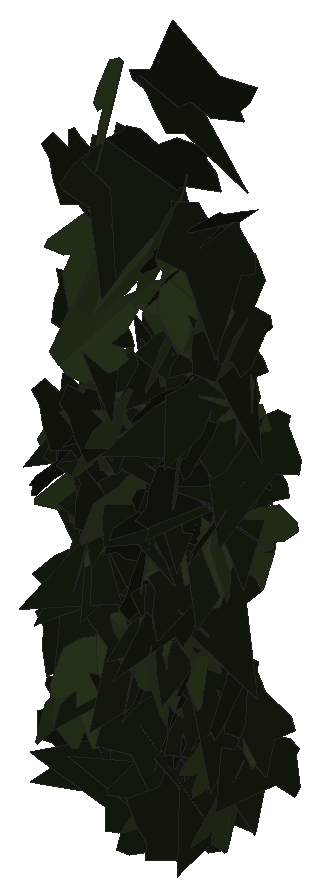
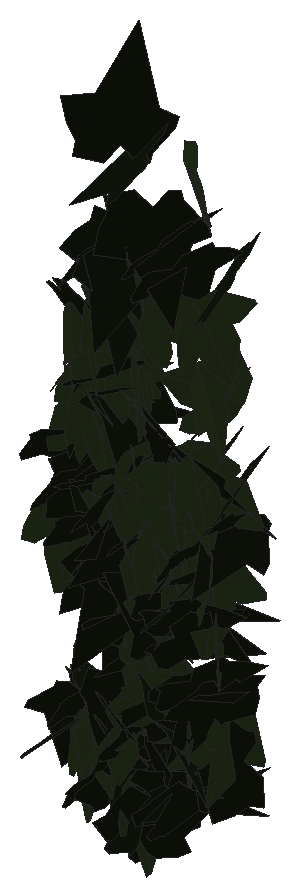
# SketchUp Ruby script. Lengths in inches.
U = 1.inch
M = Sketchup.active_model
def pt(a) = Geom::Point3d.new(a.map { |v| v * U })
def face(e, loops, mat)
  f = e.add_face(loops[0].map { |a| pt(a) })
  loops[1..].each { |l| e.add_face(l.map { |a| pt(a) }).erase! }
  f.material = f.back_material = mat if mat
  f
end
# faces: each face lists its corners as indices into pts; further lists are holes
def faces(e, pts, list, mat = nil) = list.each { |f| face(e, (f[0].is_a?(Array) ? f : [f]).map { |l| l.map { |i| pts[i] } }, mat) }
# xy, xz, yz: faces in a plane at the given z, y or x. An outline is a flat list of corners, or four numbers for a rectangle; further outlines are holes
def ring(l) = l.size == 4 ? [[l[0], l[1]], [l[2], l[1]], [l[2], l[3]], [l[0], l[3]]] : l.each_slice(2).to_a
def flat(e, list, mat, &to3) = list.each { |f| face(e, (f[0].is_a?(Array) ? f : [f]).map { |l| ring(l).map { |u, v| to3.(u, v) } }, mat) }
def xy(e, z, list, mat = nil) = flat(e, list, mat) { |x, y| [x, y, z] }
def xz(e, y, list, mat = nil) = flat(e, list, mat) { |x, z| [x, y, z] }
def yz(e, x, list, mat = nil) = flat(e, list, mat) { |y, z| [x, y, z] }
def lines(e, pts, list) = list.each { |a, b| e.add_line(pt(pts[a]), pt(pts[b])) }
# prism: a flat outline (further loops are holes) pulled along v
def prism(e, loops, v, mat = nil)
  f = face(e, loops, mat); d = Geom::Vector3d.new(v.map { |x| x * U })
  f.pushpull(f.normal.samedirection?(d) ? d.length : -d.length)
end
def box(e, o, s, mat = nil) = prism(e, [[o, [o[0] + s[0], o[1], o[2]], [o[0] + s[0], o[1] + s[1], o[2]], [o[0], o[1] + s[1], o[2]]]], [0, 0, s[2]], mat)
def at(x, y, z, deg = 0) = Geom::Transformation.translation(pt([x, y, z])) * Geom::Transformation.rotation(ORIGIN, Z_AXIS, deg.degrees)
def axes(o, x, y, z) = Geom::Transformation.new([*x, 0, *y, 0, *z, 0, *pt(o).to_a, 1])
def part(name) = M.definitions.add(name)
# library, detail: a bought-in or finely detailed component or shape, given as its bounding box
def library(name, o, s) = part(name).tap { |d| box(d.entities, o, s) }
def detail(e, o, s) = box(e.add_group.entities, o, s)
def put(e, d, t, mat = nil) = e.add_instance(d, t).tap { |i| i.material = mat if mat }
def group(e, t, mat = nil) = e.add_group.tap { |g| g.transformation = t; g.material = mat if mat }.entities
root = M.entities
M.materials.add("efeu1").color = [18, 25, 13]
M.materials.add("efeu2").color = [43, 57, 29]
c1 = part("ivyleaf_10")
p = [[0,0.5,-0.03],[-0.0625,2.02,-0.43],[-0.19,2.01,-0.46],[-0.54,1.05,-0.29],[-0.52,0.625,-0.18],[-0.83,0.76,-0.28],
  [-1.16,0.64,-0.33],[-1.15,0.33,-0.24],[-0.77,-0.39,0.02],[-0.3,-0.51,0.16],[0.04,-0.48,0.23],[-0.02,2.01,-0.4375],
  [-0.06,2.01,-0.43],[0.04,-0.49,0.23],[0.67,-0.49,0.14],[1.38,0.36,-0.2],[1.375,0.51,-0.24],[0.81,0.65,-0.19],
  [0.62,0.59,-0.15],[0.6,1.09,-0.28],[0.5,1.23,-0.31]]
faces(c1.entities,p,[[0,1,2,3,4,5,6,7,8,9,10],[11,12,0,13,14,15,16,17,18,19,20]],"efeu2")
c2 = part("ivyleaf_9")
p = [[1.54,2.16,1.25],[1.36,2.04,1.19],[-0.21,0.99,0.68],[-0.71,1.11,0.82],[-0.85,0.86,0.67],[-0.8,0.17,0.21],
  [-0.9,-0.01,0.1],[-0.67,-0.16,-0.02],[-0.08,-0.08,-0.05],[-0.03,-0.6,-0.4],[0.65,-0.88,-0.66],[0.83,-0.6,-0.49],
  [1.29,-0.42,-0.43],[1.8125,-0.07,-0.26],[1.21,0.44,0.15]]
faces(c2.entities,p,[[0,1,2,3,4,5,6,7,8,9,10,11,12,13,14]],"efeu1")
put(root,c1,axes([28.08,223.25,228.54],[-0.03699,-0.29096,0.40494],[0.03888,0.40313,0.29321],[-0.49711,0.05318,-0.0072]))
put(root,c2,axes([29.68,223.84,228.08],[-0.38606,-0.14286,0.28381],[-0.22488,-0.19267,-0.40287],[0.22447,-0.43871,0.08452]))
put(root,c1,axes([28.625,223.375,226.82],[-0.19709,-0.38444,-0.25172],[0.11734,0.22271,-0.43201],[0.44429,-0.22936,0.00243]))
put(root,c2,axes([29.57,223.75,230.38],[0.03682,-0.49858,0.00801],[-0.01166,-0.00889,-0.49978],[0.49851,0.03662,-0.01228]))
put(root,c1,axes([29.63,223.53,229.73],[0.23294,0.05076,-0.4395],[-0.44042,0.07385,-0.22489],[0.04208,0.4919,0.07912]))
put(root,c2,axes([29.31,223.67,225.79],[-0.46975,0.11695,-0.12514],[0.11369,-0.06035,-0.48315],[-0.12811,-0.48237,0.0301]))
put(root,c1,axes([29.58,223.56,226.44],[0.31812,0.02424,-0.38498],[-0.38501,0.0506,-0.31497],[0.02369,0.49684,0.05086]))
put(root,c1,axes([28,223.75,229.83],[-0.10963,-0.44335,0.20352],[0.02476,-0.21338,-0.4515],[0.4872,-0.08892,0.06874]))
put(root,c2,axes([28.43,223.86,225.8],[-0.38779,-0.18037,0.259],[-0.21037,-0.15816,-0.42512],[0.23529,-0.43869,0.04678]))
put(root,c1,axes([28.09,223.55,224.47],[0.28723,0.40918,-0.00836],[-0.00572,-0.00621,-0.49993],[-0.40923,0.28728,0.00111]))
put(root,c1,axes([28.56,223.92,229.79],[-0.00929,-0.24651,0.43491],[0.05978,-0.43241,-0.24382],[0.49633,0.04746,0.03751]))
put(root,c1,axes([28.18,223.73,231.8125],[0.33389,-0.33576,0.16058],[0.10981,-0.11725,-0.47349],[0.35561,0.35145,-0.00456]))
put(root,c2,axes([29.52,223.27,227.61],[-0.34745,0.34738,-0.09278],[-0.08278,0.04827,0.49073],[0.34989,0.35637,0.02397]))
put(root,c2,axes([29.55,223.56,225.98],[-0.15467,-0.18929,-0.43617],[0.31494,0.30284,-0.2431],[0.35621,-0.34994,0.02555]))
put(root,c2,axes([27.58,223.59,227.61],[0.29977,-0.38606,-0.10531],[-0.04876,0.09536,-0.48839],[0.39719,0.30309,0.01952]))
put(root,c2,axes([29.49,223.36,226.86],[-0.04579,-0.15221,0.47406],[0.41961,0.24446,0.11902],[-0.26802,0.40874,0.10534]))
put(root,c1,axes([28.375,223.47,227.625],[-0.02489,-0.45557,-0.20453],[0.01667,0.20391,-0.45623],[0.4991,-0.02953,0.00504]))
put(root,c1,axes([27.82,223.375,224.1],[-0.04349,-0.38433,-0.31686],[0.04132,0.31418,-0.38676],[0.49639,-0.05982,0.00443]))
put(root,c1,axes([29.02,223.48,224.94],[0.02898,0.11506,0.48572],[-0.49645,0.05726,0.01606],[-0.05193,-0.4832,0.11756]))
put(root,c2,axes([28.19,223.74,226.5625],[0.14925,-0.47656,-0.02477],[-0.00906,0.02312,-0.49938],[0.47712,0.14952,-0.00173]))
put(root,c2,axes([28.54,223.94,230.75],[-0.11137,-0.45827,0.16608],[0.01845,-0.1742,-0.46831],[0.48709,-0.09818,0.05571]))
put(root,c1,axes([29.16,223.38,224.86],[-0.15807,0.41024,0.23816],[-0.10102,0.21616,-0.4394],[-0.46348,-0.18702,0.01455]))
put(root,c1,axes([29.34,223.46,227.71],[0.25601,-0.34801,-0.25168],[-0.0366,0.27426,-0.41646],[0.42792,0.23166,0.11495]))
put(root,c2,axes([27.68,223.47,223.73],[0.19179,0.06943,-0.4565],[0.32704,0.32853,0.18737],[0.32597,-0.37047,0.08061]))
put(root,c1,axes([29.17,223.59,230.6],[0.1301,-0.46536,-0.12851],[-0.04314,0.12136,-0.48313],[0.48085,0.1368,-0.00858]))
put(root,c2,axes([27.97,223.53,227.78],[0.33189,-0.30641,-0.21438],[-0.1141,0.18999,-0.4482],[0.35613,0.34643,0.05619]))
put(root,c2,axes([28.35,223.75,227.71],[-0.48671,0.04347,0.10593],[-0.10596,0.0043,-0.48862],[-0.04339,-0.49809,0.00503]))
put(root,c1,axes([29.34,223.54,225.35],[-0.46437,0.08562,0.1644],[-0.16275,0.02391,-0.47217],[-0.08872,-0.49203,0.00566]))
put(root,c1,axes([27.98,223.57,227.4],[-0.45551,-0.18464,-0.09177],[0.08744,0.02854,-0.49147],[0.18673,-0.46378,0.00629]))
put(root,c2,axes([29.03,223.88,227.375],[-0.0155,-0.49912,0.02533],[0.00645,-0.02554,-0.49931],[0.49972,-0.01516,0.00723]))
put(root,c2,axes([29.91,223.57,227.04],[-0.29347,0.40056,-0.05854],[0.0401,-0.04319,-0.49651],[-0.40282,-0.29612,-0.00678]))
put(root,c2,axes([29.46,223.51,222.75],[-0.2807,-0.26972,0.31378],[0.22438,0.21935,0.38928],[-0.34765,0.35936,-0.00211]))
put(root,c1,axes([27.9,223.32,224.1],[0.04396,-0.15904,-0.47199],[0.20573,0.43731,-0.1282],[0.45359,-0.18294,0.10389]))
put(root,c1,axes([29.13,223.78,229.5],[0.40583,-0.16069,0.24389],[0.23915,-0.05683,-0.4354],[0.16765,0.47005,0.03073]))
put(root,c1,axes([29.45,223.375,229.76],[0.00652,0.37111,0.33501],[0.01919,0.33461,-0.37104],[-0.49959,0.01769,-0.00988]))
put(root,c2,axes([29.24,223.8,231.95],[0.44556,0.00718,0.22677],[-0.22689,0.01595,0.44527],[-0.00084,-0.49969,0.01747]))
put(root,c2,axes([28.6875,223.71,226.79],[0.10229,-0.44712,-0.19905],[0.01685,0.20645,-0.45508],[0.48914,0.08639,0.0573]))
put(root,c1,axes([29.92,223.63,223.35],[0.05686,-0.47774,-0.13612],[-0.02185,0.13447,-0.48108],[0.49628,0.06065,-0.00559]))
put(root,c1,axes([29.34,223.66,228.9],[-0.43427,-0.02447,0.2466],[-0.24369,-0.04824,-0.43392],[0.04503,-0.49707,0.02998]))
put(root,c1,axes([29.31,223.64,225.03],[0.3868,-0.17122,-0.26658],[-0.22455,0.14866,-0.42128],[0.22352,0.44563,0.03811]))
put(root,c2,axes([27.77,223.29,227.04],[0.11803,0.40788,0.26402],[0.05772,0.258,-0.42439],[-0.48243,0.13066,0.01382]))
put(root,c2,axes([29.4375,223.99,228.66],[-0.26278,-0.42291,0.04577],[0.01563,-0.06337,-0.49572],[0.42509,-0.2591,0.04653]))
put(root,c2,axes([29.69,223.83,229.01],[0.20689,-0.45519,-0.00031],[0.00004,0.00036,-0.5],[0.45519,0.20689,0.00018]))
put(root,c2,axes([28.47,223.99,222.85],[-0.21599,0.03933,0.44922],[-0.37335,-0.29494,-0.15369],[0.2529,-0.40183,0.15677]))
put(root,c2,axes([28.97,223.75,226.94],[0.30088,-0.2774,0.28727],[0.30167,-0.07779,-0.39108],[0.26166,0.40865,0.12055]))
put(root,c2,axes([28.92,223.29,226.75],[-0.04651,0.20349,-0.45435],[-0.10338,0.44243,0.20873],[0.48698,0.11336,0.00092]))
put(root,c2,axes([28.76,223.85,223.96],[-0.05654,-0.479,-0.13177],[0.02097,0.1302,-0.48229],[0.49635,-0.06007,0.00537]))
put(root,c1,axes([29.84,223.53,226.56],[-0.24779,0.19551,0.38778],[-0.37362,0.13161,-0.3051],[-0.22137,-0.44097,0.08087]))
put(root,c2,axes([27.71,223.93,228.74],[0.14696,-0.46938,0.08991],[0.02282,-0.08706,-0.49183],[0.47737,0.14866,-0.00417]))
put(root,c1,axes([28.5,223.71,226.47],[-0.13013,-0.02101,0.48231],[0.47778,0.06603,0.13178],[-0.06923,0.49518,0.00289]))
put(root,c2,axes([28.27,223.97,230.56],[-0.17347,-0.4689,0.00634],[0.00007,-0.00678,-0.49995],[0.46894,-0.17346,0.00242]))
put(root,c2,axes([29.13,223.5625,226.9375],[0.30608,-0.27307,-0.28592],[-0.11824,0.28182,-0.39572],[0.37727,0.30986,0.10794]))
put(root,c1,axes([28.71,223.64,226.32],[0.29039,-0.32934,-0.23918],[-0.0969,0.22943,-0.43356],[0.39533,0.29815,0.06942]))
put(root,c1,axes([29.7,223.83,228.02],[-0.35163,-0.34439,0.08803],[-0.0101,-0.1141,-0.4867],[0.35532,-0.34406,0.07328]))
put(root,c1,axes([28.42,223.69,227.43],[-0.42529,0.10999,0.23882],[-0.24805,-0.01725,-0.43379],[-0.08718,-0.48745,0.06924]))
put(root,c2,axes([27.53,223.78,230.65],[0.31607,-0.3763,-0.09218],[-0.05534,0.0739,-0.4914],[0.38346,0.32084,0.00506]))
put(root,c2,axes([29.4,224.11,223.25],[-0.10205,-0.44769,0.19788],[-0.02796,-0.19647,-0.45893],[0.48868,-0.10473,0.01507]))
put(root,c2,axes([30.05,223.84,229.52],[-0.48833,0.10461,0.02429],[-0.02079,0.01884,-0.49921],[-0.10536,-0.48857,-0.01405]))
put(root,c2,axes([29.34,223.5,228.43],[0.04801,0.49682,0.02941],[-0.04996,0.03421,-0.49632],[-0.49518,0.04472,0.05293]))
put(root,c2,axes([27.86,224.04,226.92],[-0.05495,-0.49291,0.06337],[-0.00348,-0.06337,-0.49596],[0.49696,-0.05495,0.00353]))
put(root,c1,axes([28.99,223.76,227.47],[-0.44336,-0.22323,0.06002],[-0.05369,-0.02682,-0.49638],[0.22483,-0.4466,-0.00019]))
put(root,c1,axes([28.92,223.79,222.99],[-0.0059,-0.49814,-0.04271],[0.00647,0.04263,-0.49814],[0.49992,-0.00643,0.00594]))
put(root,c1,axes([29.05,223.67,228.95],[0.13628,-0.42778,-0.22007],[-0.0458,0.21615,-0.44853],[0.47889,0.14241,0.01973]))
put(root,c1,axes([27.86,223.88,229.05],[0.1205,-0.48266,0.0502],[0.02552,-0.04535,-0.49728],[0.48459,0.12241,0.01371]))
put(root,c2,axes([28.6,224.01,223.23],[-0.40516,-0.04595,0.28937],[-0.27704,-0.10063,-0.40388],[0.09535,-0.48761,0.05608]))
put(root,c2,axes([29.4375,224.16,227.33],[-0.34427,-0.33144,0.14706],[0.00859,-0.21019,-0.45359],[0.3625,-0.30979,0.15042]))
put(root,c2,axes([29.1,224.08,225.52],[-0.17473,-0.46702,0.03692],[-0.02346,-0.03063,-0.49851],[0.46789,-0.17594,-0.01121]))
put(root,c2,axes([29.27,223.93,225.64],[-0.49736,0.03523,0.0373],[-0.03709,0.00421,-0.4986],[-0.03545,-0.49874,-0.00157]))
put(root,c2,axes([29.53,224.07,226.74],[-0.1839,-0.46478,-0.01277],[0.00817,0.01049,-0.49982],[0.46488,-0.18404,0.00374]))
put(root,c2,axes([28.46,224.19,224.63],[-0.23779,-0.39899,0.18511],[-0.05358,-0.18259,-0.46238],[0.43656,-0.23973,0.04408]))
put(root,c2,axes([28.06,224.18,224.53],[-0.29104,-0.3745,0.15827],[-0.05554,-0.15619,-0.47172],[0.40276,-0.29216,0.04932]))
put(root,c1,axes([28.53,224.05,226.55],[-0.26703,-0.28379,0.3133],[-0.13492,-0.29398,-0.38128],[0.40062,-0.28817,0.08042]))
put(root,c1,axes([29.23,223.77,226.23],[-0.46554,0.18038,-0.02707],[0.02434,-0.01211,-0.49926],[-0.18076,-0.46617,0.00249]))
put(root,c1,axes([29.54,223.96,223.76],[0.07787,-0.48582,0.08899],[0.01266,-0.0881,-0.49201],[0.49374,0.07888,-0.00142]))
put(root,c2,axes([29.53,223.83,227.32],[0.14512,0.33048,-0.34601],[-0.14288,-0.31514,-0.36093],[-0.45665,0.20363,0.00297]))
put(root,c2,axes([28.82,224.04,222.53],[-0.07103,0.06599,0.49051],[-0.47605,-0.14466,-0.04947],[0.13539,-0.47404,0.08338]))
put(root,c2,axes([29.36,223.52,230.3],[0.16166,0.4641,0.09208],[-0.01215,0.10135,-0.48947],[-0.47299,0.15601,0.04405]))
put(root,c2,axes([29.39,223.55,230],[-0.01405,0.48555,0.11851],[-0.01201,0.11819,-0.48568],[-0.49966,-0.0165,0.00834]))
put(root,c1,axes([29.59,223.85,229.45],[0.09952,-0.4845,-0.07316],[0.03026,0.08059,-0.49253],[0.48906,0.0936,0.04536]))
put(root,c1,axes([28.82,224.02,224.39],[0.22625,0.22266,-0.38631],[-0.34002,-0.19407,-0.311],[-0.28844,0.40343,0.06361]))
put(root,c2,axes([29.85,224.12,227.85],[-0.21324,-0.45183,-0.01948],[0.01948,0.01234,-0.49947],[0.45183,-0.21377,0.01234]))
put(root,c2,axes([28.21,224.16,226.18],[-0.28637,-0.40656,0.05197],[-0.01727,-0.05137,-0.49705],[0.4095,-0.28648,0.01537]))
put(root,c1,axes([27.82,223.75,225.95],[0.19702,-0.36809,-0.27513],[-0.09887,0.25838,-0.41649],[0.44878,0.21852,0.02903]))
put(root,c2,axes([28.84,223.88,231.91],[0.36064,-0.3442,-0.03826],[0.03301,0.08916,-0.49088],[0.34474,0.35154,0.08703]))
put(root,c2,axes([28,224.24,225.66],[-0.30813,-0.33131,0.21281],[-0.14676,-0.15412,-0.45245],[0.3654,-0.34129,-0.00226]))
put(root,c1,axes([27.8125,223.89,226.42],[-0.37709,-0.32834,-0.0005],[0.00069,-0.00003,-0.5],[0.32834,-0.37709,0.00048]))
put(root,c1,axes([28.32,223.84,224.48],[0.29969,-0.35284,-0.18891],[-0.08485,0.17463,-0.46077],[0.39113,0.30823,0.0448]))
put(root,c2,axes([29.67,224.09,227.34],[-0.00651,-0.49694,-0.05483],[-0.0024,0.05486,-0.49698],[0.49995,-0.0062,-0.0031]))
put(root,c1,axes([29.77,223.97,228.35],[0.42472,-0.2638,-0.00506],[0.00072,0.01076,-0.49988],[0.26385,0.42461,0.00952]))
put(root,c2,axes([28.73,223.83,231.125],[0.23888,0.29106,-0.32897],[-0.21924,-0.24549,-0.37639],[-0.38062,0.32407,0.01033]))
put(root,c2,axes([27.8,224.2,225.11],[-0.27944,-0.41007,0.06124],[-0.03429,-0.05075,-0.49623],[0.4132,-0.28154,0.00024]))
put(root,c2,axes([29,223.68,227.86],[-0.03252,0.06263,0.49499],[-0.22984,0.4384,-0.07057],[-0.44285,-0.23213,0.00028]))
put(root,c1,axes([29.16,224.01,226.85],[0.34135,-0.362,0.04939],[0.06013,-0.01101,-0.49625],[0.36037,0.34473,0.03602]))
put(root,c2,axes([28.73,223.64,225.41],[0.04662,-0.12457,0.48198],[0.25517,0.42164,0.08429],[-0.42745,0.23812,0.10289]))
put(root,c2,axes([28.61,223.75,224.32],[-0.26656,0.39518,0.15091],[-0.07581,0.13086,-0.47658],[-0.41617,-0.27696,-0.00985]))
put(root,c2,axes([29.04,224.07,227.28],[0.10096,-0.4813,-0.09031],[0.00064,0.09234,-0.4914],[0.4897,0.09911,0.01926]))
put(root,c1,axes([28.93,223.92,227.67],[0.25715,-0.41557,-0.10572],[-0.00233,0.12191,-0.4849],[0.4288,0.24987,0.06076]))
put(root,c1,axes([28.29,223.93,226.03],[0.3248,0.37986,0.01463],[0.01242,0.00862,-0.49977],[-0.37994,0.32501,-0.00384]))
put(root,c2,axes([28.96,223.67,223.45],[-0.0488,0.11542,0.48404],[-0.20603,0.43803,-0.12522],[-0.45296,-0.21168,0.00481]))
put(root,c1,axes([28.36,223.89,227.36],[0.35723,-0.30763,-0.16657],[-0.07296,0.16733,-0.46549],[0.34214,0.35688,0.07466]))
put(root,c1,axes([29.39,223.96,228.73],[-0.41333,-0.28129,0.00546],[0.01772,-0.03571,-0.49841],[0.28079,-0.41182,0.03949]))
put(root,c1,axes([27.9,224.02,227.87],[0.00415,-0.49952,0.02149],[-0.00032,-0.02149,-0.49954],[0.49998,0.00413,-0.00049]))
put(root,c1,axes([28.37,224.21,226.87],[-0.07146,-0.4067,0.28194],[0.10045,-0.29085,-0.3941],[0.48456,0.00031,0.12328]))
put(root,c1,axes([29.91,223.89,229.19],[0.13626,-0.45305,-0.16179],[-0.03377,0.15873,-0.47293],[0.47989,0.13981,0.01266]))
put(root,c2,axes([29.62,224.02,224.1875],[-0.18246,-0.35836,-0.29713],[0.14821,0.25782,-0.40195],[0.4413,-0.23475,0.01214]))
put(root,c2,axes([29.6,224.06,224.48],[-0.41894,0.20368,-0.18167],[0.14792,-0.11025,-0.46472],[-0.22936,-0.44312,0.03213]))
put(root,c1,axes([28.79,224.02,227.64],[-0.04561,-0.49746,0.0212],[-0.00412,-0.02091,-0.49955],[0.4979,-0.04574,-0.00219]))
put(root,c2,axes([27.98,224.28,226.26],[0.02671,-0.44212,0.23199],[0.08562,-0.22483,-0.43832],[0.49189,0.06314,0.0637]))
put(root,c1,axes([28.6,224.24,227.49],[-0.22884,-0.27856,0.34647],[-0.06984,-0.36231,-0.33742],[0.43904,-0.20283,0.12691]))
put(root,c2,axes([29.25,224.11,224.66],[-0.23394,0.25159,-0.36328],[0.24325,-0.26985,-0.34353],[-0.36892,-0.33747,0.00386]))
put(root,c2,axes([28.82,224.04,228.48],[-0.47067,0.16822,-0.01296],[0.00787,-0.01648,-0.49967],[-0.16853,-0.47056,0.01286]))
put(root,c2,axes([29.39,224.25,224.48],[-0.03915,-0.49262,0.07609],[-0.00569,-0.07588,-0.49418],[0.49843,-0.03956,0.00034]))
put(root,c2,axes([27.65,223.89,224.85],[0.07366,-0.3603,-0.33876],[-0.04159,0.33677,-0.36722],[0.49279,0.08227,0.01965]))
put(root,c1,axes([27.78,224.06,226.67],[-0.31148,0.29013,-0.2623],[0.17499,-0.19651,-0.42516],[-0.3498,-0.35666,0.02088]))
put(root,c1,axes([29.42,224.04,228.375],[-0.1361,-0.48065,0.0213],[0.00344,-0.02311,-0.49945],[0.48111,-0.1358,0.00959]))
put(root,c2,axes([28.65,223.71,226.95],[0.43744,0.20532,0.1284],[0.10223,0.08376,-0.48222],[-0.21953,0.44814,0.0313]))
put(root,c2,axes([29.83,224.39,223.72],[-0.18207,-0.37438,0.27693],[0.04871,-0.31103,-0.38845],[0.46312,-0.11447,0.14973]))
put(root,c1,axes([29.92,223.95,226.64],[-0.32027,-0.37814,-0.06657],[0.03167,0.06037,-0.49533],[0.38265,-0.3215,-0.01472]))
put(root,c2,axes([28.5625,224.25,222.95],[0.11581,-0.28067,0.39725],[0.23613,-0.32457,-0.29816],[0.42524,0.25667,0.05737]))
put(root,c1,axes([28.52,224.09,226.62],[0.42939,-0.21294,0.14241],[0.14318,-0.03098,-0.47806],[0.21242,0.45133,0.03438]))
put(root,c2,axes([28.04,224.26,225.98],[-0.43061,-0.25101,0.0396],[-0.02817,-0.03029,-0.49829],[0.25255,-0.43137,0.01194]))
put(root,c2,axes([27.96,224.3125,225.91],[0.03543,-0.46071,0.19104],[0.05824,-0.18639,-0.46029],[0.49533,0.05487,0.04045]))
put(root,c2,axes([29.08,223.74,226.01],[0.37939,0.32552,0.00984],[0.00753,0.00634,-0.4999],[-0.32559,0.37946,-0.0001]))
put(root,c1,axes([29.08,224.09,223.92],[-0.17378,-0.01515,-0.46859],[0.43467,-0.19246,-0.15498],[-0.17568,-0.46122,0.08006]))
put(root,c2,axes([29.43,224.17,224.37],[-0.45238,-0.00877,-0.21278],[0.21295,-0.02353,-0.45177],[-0.00208,-0.49937,0.02502]))
put(root,c1,axes([29.18,224.07,226.89],[0.4995,-0.01663,0.0149],[0.0149,-0.00022,-0.49978],[0.01663,0.49972,0.00027]))
